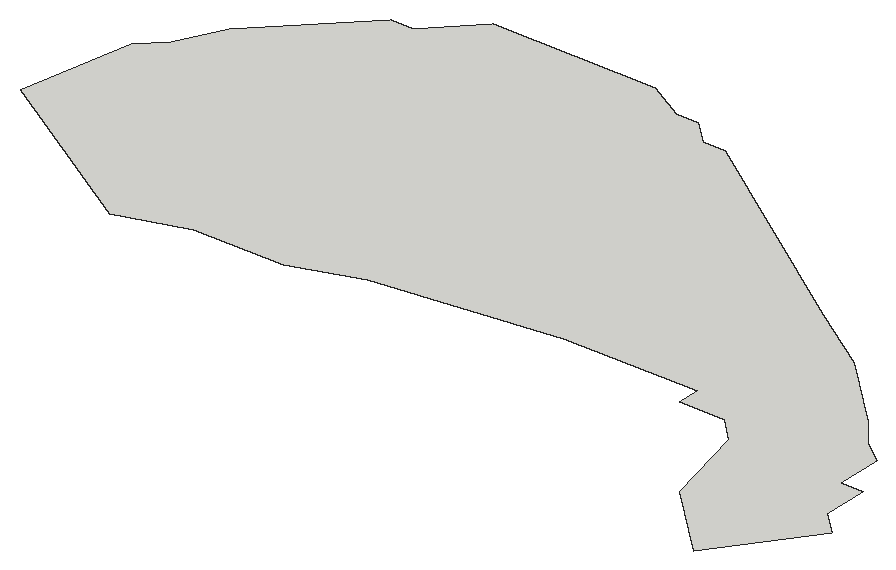
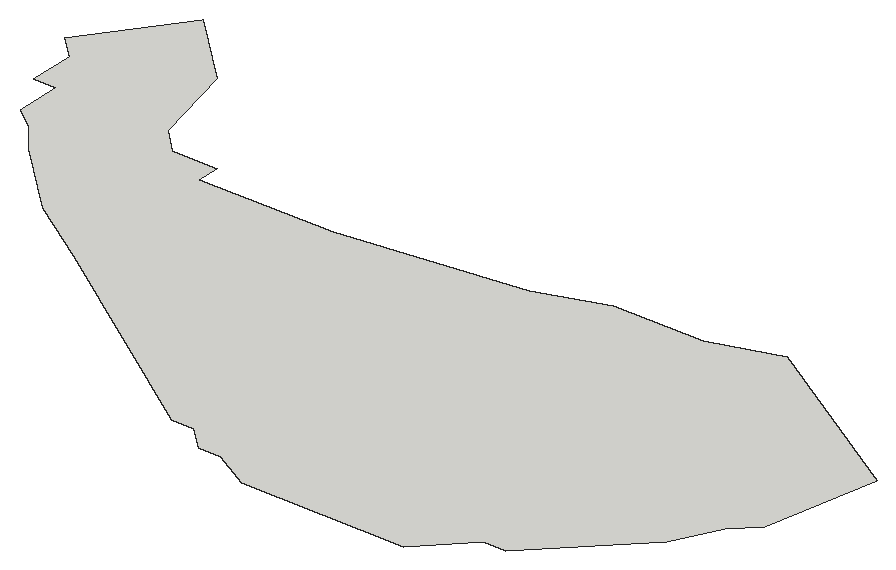
# SketchUp Ruby script. Lengths in inches.
U = 1.inch
M = Sketchup.active_model
def pt(a) = Geom::Point3d.new(a.map { |v| v * U })
def face(e, loops, mat)
  f = e.add_face(loops[0].map { |a| pt(a) })
  loops[1..].each { |l| e.add_face(l.map { |a| pt(a) }).erase! }
  f.material = f.back_material = mat if mat
  f
end
# faces: each face lists its corners as indices into pts; further lists are holes
def faces(e, pts, list, mat = nil) = list.each { |f| face(e, (f[0].is_a?(Array) ? f : [f]).map { |l| l.map { |i| pts[i] } }, mat) }
# xy, xz, yz: faces in a plane at the given z, y or x. An outline is a flat list of corners, or four numbers for a rectangle; further outlines are holes
def ring(l) = l.size == 4 ? [[l[0], l[1]], [l[2], l[1]], [l[2], l[3]], [l[0], l[3]]] : l.each_slice(2).to_a
def flat(e, list, mat, &to3) = list.each { |f| face(e, (f[0].is_a?(Array) ? f : [f]).map { |l| ring(l).map { |u, v| to3.(u, v) } }, mat) }
def xy(e, z, list, mat = nil) = flat(e, list, mat) { |x, y| [x, y, z] }
def xz(e, y, list, mat = nil) = flat(e, list, mat) { |x, z| [x, y, z] }
def yz(e, x, list, mat = nil) = flat(e, list, mat) { |y, z| [x, y, z] }
def lines(e, pts, list) = list.each { |a, b| e.add_line(pt(pts[a]), pt(pts[b])) }
# prism: a flat outline (further loops are holes) pulled along v
def prism(e, loops, v, mat = nil)
  f = face(e, loops, mat); d = Geom::Vector3d.new(v.map { |x| x * U })
  f.pushpull(f.normal.samedirection?(d) ? d.length : -d.length)
end
def box(e, o, s, mat = nil) = prism(e, [[o, [o[0] + s[0], o[1], o[2]], [o[0] + s[0], o[1] + s[1], o[2]], [o[0], o[1] + s[1], o[2]]]], [0, 0, s[2]], mat)
def at(x, y, z, deg = 0) = Geom::Transformation.translation(pt([x, y, z])) * Geom::Transformation.rotation(ORIGIN, Z_AXIS, deg.degrees)
def axes(o, x, y, z) = Geom::Transformation.new([*x, 0, *y, 0, *z, 0, *pt(o).to_a, 1])
def part(name) = M.definitions.add(name)
# library, detail: a bought-in or finely detailed component or shape, given as its bounding box
def library(name, o, s) = part(name).tap { |d| box(d.entities, o, s) }
def detail(e, o, s) = box(e.add_group.entities, o, s)
def put(e, d, t, mat = nil) = e.add_instance(d, t).tap { |i| i.material = mat if mat }
def group(e, t, mat = nil) = e.add_group.tap { |g| g.transformation = t; g.material = mat if mat }.entities
root = M.entities
xy(root,0,[[15.515,360.083,15.525,360.083,15.526,360.084,15.527,360.084,15.532,360.086,15.544,360.095,15.55,360.101,15.551,360.103,15.553,360.105,15.555,360.109,15.555,360.112,15.556,360.114,15.556,360.116,15.557,360.118,15.557,360.125,15.551,360.149,15.548,360.156,15.544,360.164,15.53,360.186,15.521,360.197,15.512,360.207,15.489,360.229,15.464,360.249,15.364,360.316,15.351,360.323,15.339,360.329,15.325,360.334,15.312,360.338,15.298,360.342,15.292,360.343,15.274,360.343,15.256,360.34,15.251,360.338,15.245,360.336,15.234,360.331,15.212,360.317,15.203,360.31,15.193,360.301,15.182,360.289,15.172,360.276,15.162,360.262,15.154,360.247,15.147,360.232,15.144,360.223,15.144,360.206,15.145,360.203,15.145,360.2,15.147,360.197,15.149,360.191,15.151,360.1875,15.153,360.185,15.155,360.182,15.165,360.172,15.18,360.163,15.195,360.157,15.201,360.156,15.206,360.155,15.212,360.154,15.218,360.154,15.252,360.156,15.287,360.16,15.321,360.167,15.396,360.181,15.407,360.182,15.429,360.182,15.439,360.18,15.45,360.178,15.458,360.176,15.462,360.174,15.466,360.173,15.469,360.17,15.473,360.168,15.476,360.166,15.482,360.16,15.485,360.158,15.486,360.155,15.488,360.152,15.49,360.15,15.495,360.135,15.495,360.121,15.497,360.107,15.499,360.1,15.499,360.099,15.501,360.095,15.501,360.094,15.502,360.092,15.504,360.091,15.505,360.09,15.506,360.088,15.507,360.087,15.509,360.086,15.51,360.085,15.511,360.085,15.513,360.084,15.514,360.084]])
